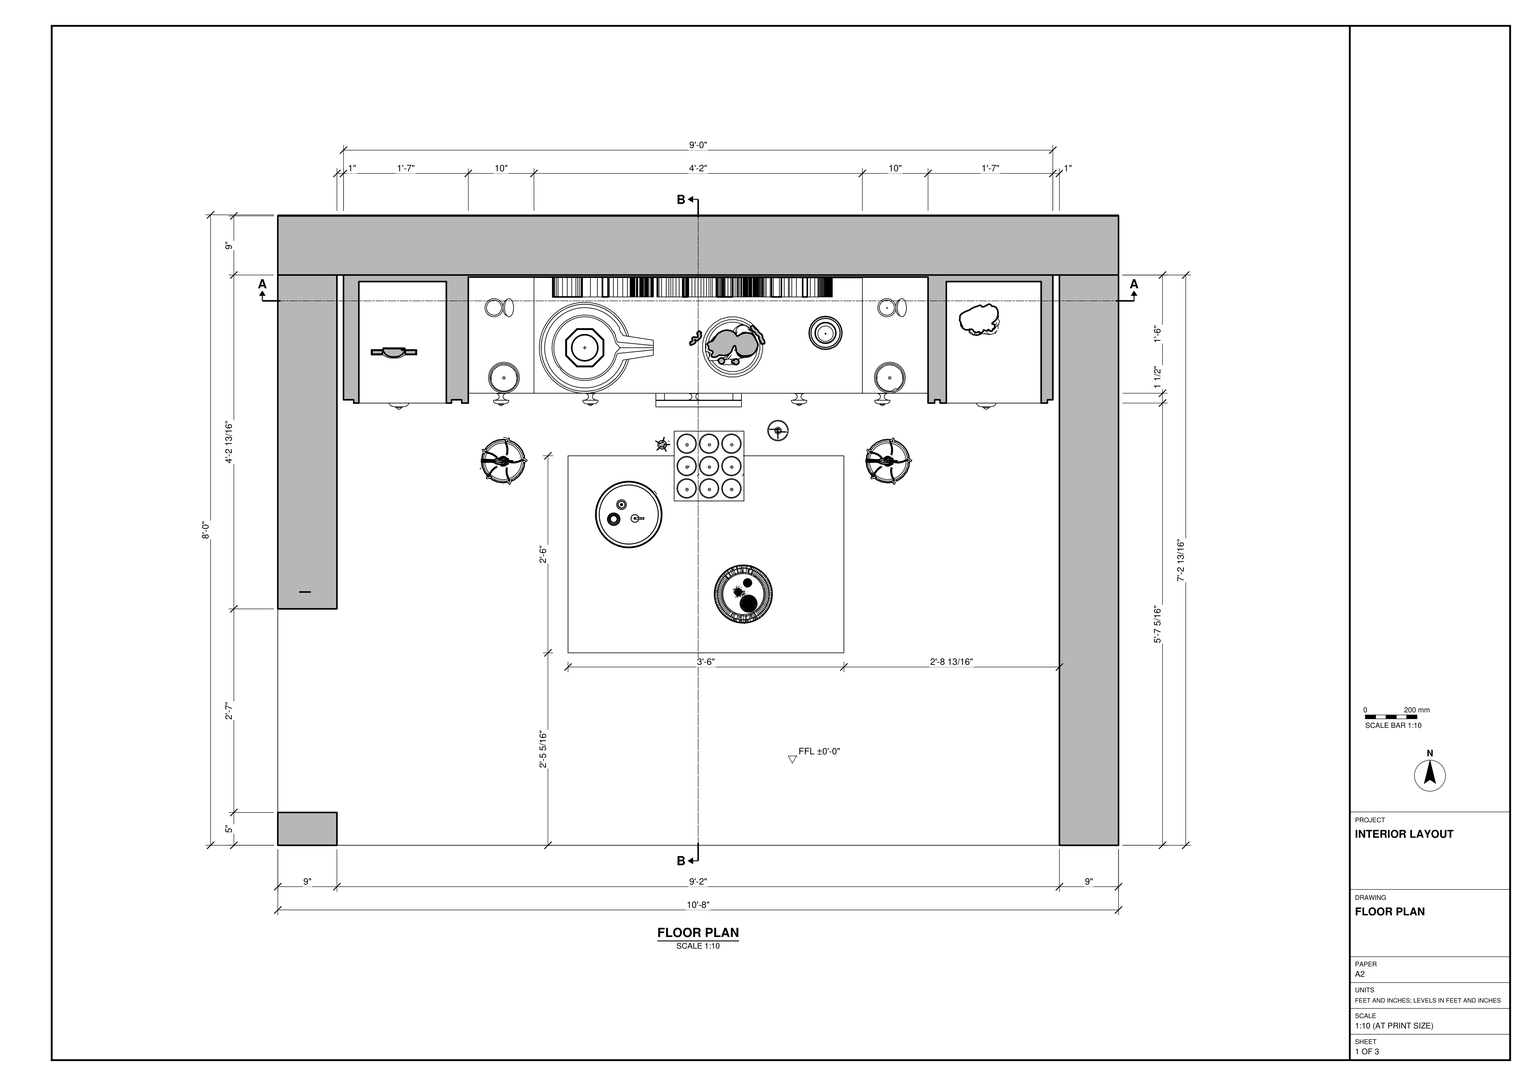
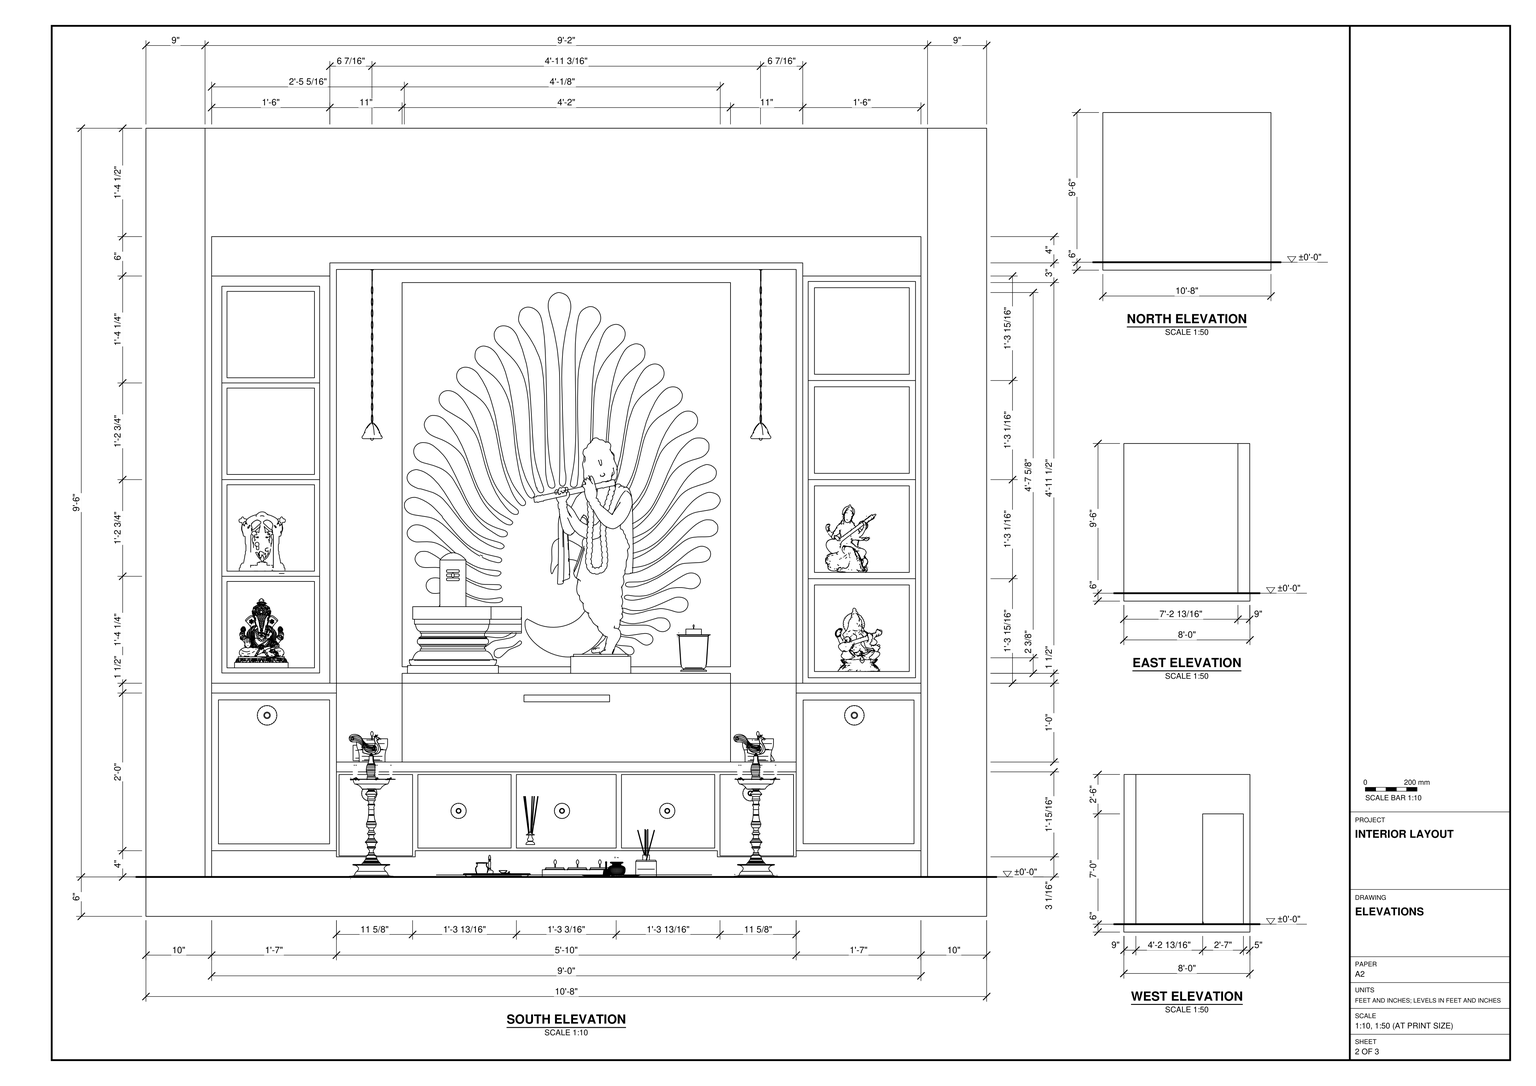
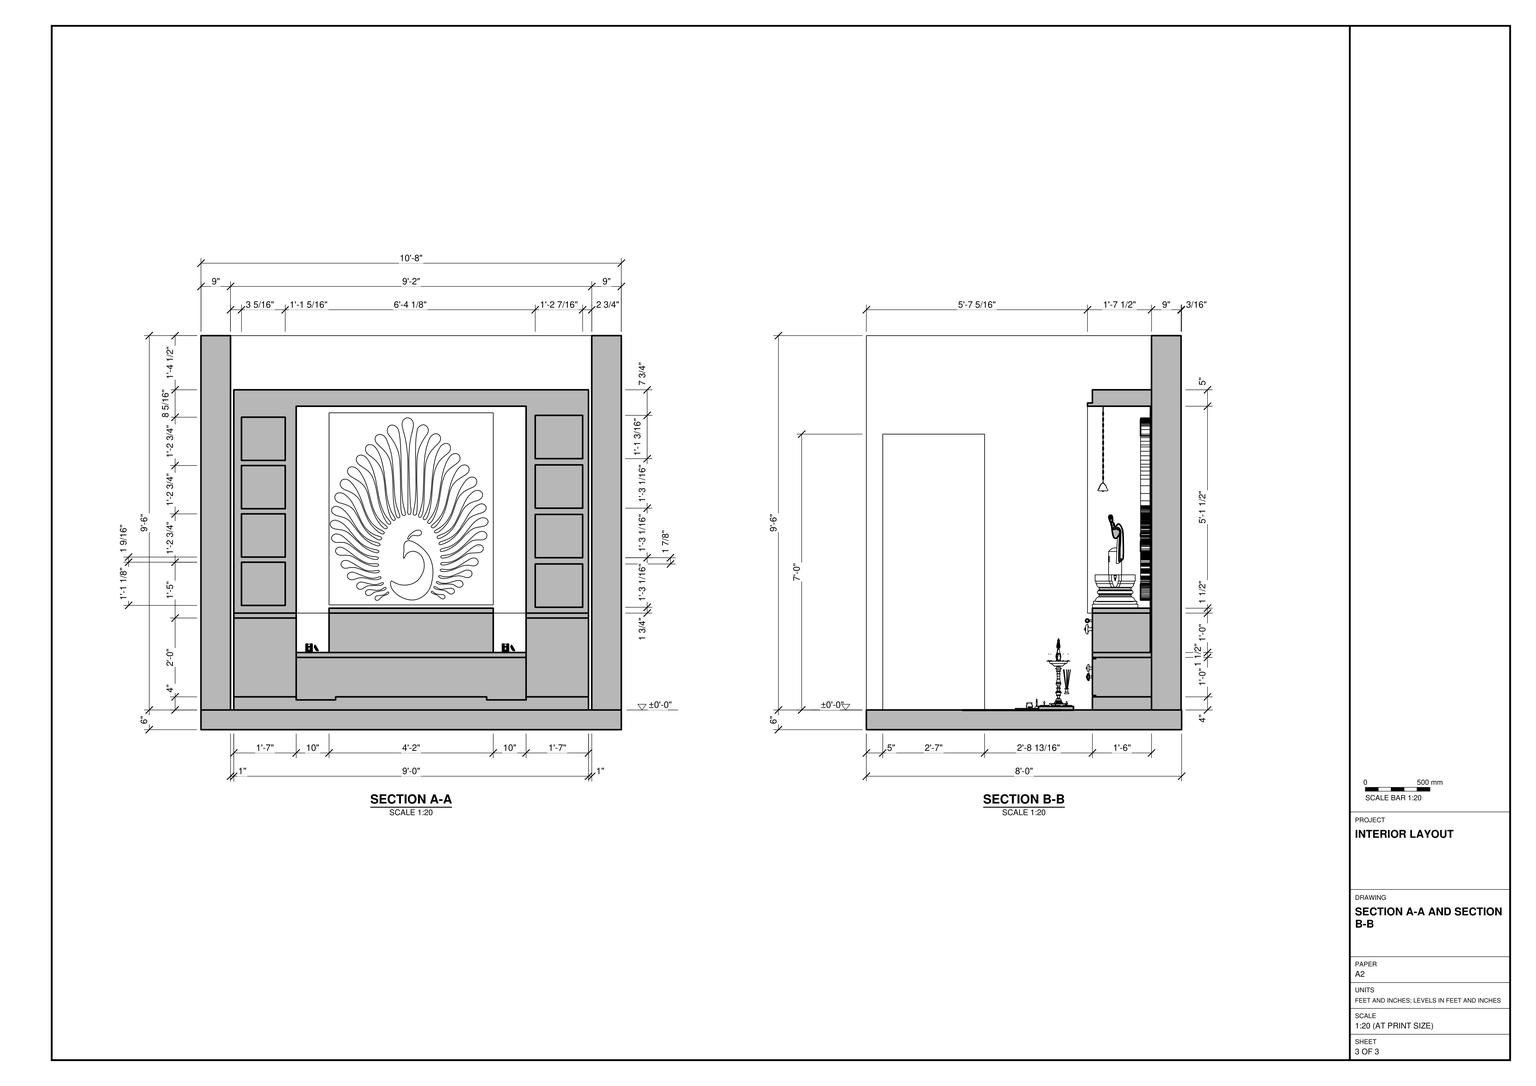
Build the prayer room in SketchUp from task_files/diagram_01.pdf. Work in feet and inches. Set the finished floor at ±0'-0". The room shell measures 10'-8" across the shrine wall and 8'-0" from front to back, with an overall height of 10'-0" from the underside of the slab. Model the 6" floor slab and the 9" walls. Leave the south side open as drawn and form the doorway near the south end of the west wall, retaining the short wall return beyond it.

Use the south elevation for the joinery fronts and the sections for their depths and changes in height. Build the 9'-0" shrine unit against the north wall. At each end, place a stack of display compartments above a lower cupboard. Between the cupboards, model the low storage run, the narrower raised display cabinet and the feature panel with its radiating motif. Include the headpiece that spans the display. Place figures on the raised surface and in the lower display compartments. Arrange the hanging ornaments, standing lamps and floor accessories using the plan and elevation together. Decor and loose items may be any suitable library components.

Keep the walls, floor slab and each furniture or joinery piece in separate groups or components, and use components for repeated parts. Save one SketchUp model as output_files/prayer_room_with_a_built_in_shrine.skp.

# SketchUp Ruby script. Lengths in inches.
U = 1.inch
M = Sketchup.active_model
def pt(a) = Geom::Point3d.new(a.map { |v| v * U })
def face(e, loops, mat)
  f = e.add_face(loops[0].map { |a| pt(a) })
  loops[1..].each { |l| e.add_face(l.map { |a| pt(a) }).erase! }
  f.material = f.back_material = mat if mat
  f
end
# faces: each face lists its corners as indices into pts; further lists are holes
def faces(e, pts, list, mat = nil) = list.each { |f| face(e, (f[0].is_a?(Array) ? f : [f]).map { |l| l.map { |i| pts[i] } }, mat) }
# xy, xz, yz: faces in a plane at the given z, y or x. An outline is a flat list of corners, or four numbers for a rectangle; further outlines are holes
def ring(l) = l.size == 4 ? [[l[0], l[1]], [l[2], l[1]], [l[2], l[3]], [l[0], l[3]]] : l.each_slice(2).to_a
def flat(e, list, mat, &to3) = list.each { |f| face(e, (f[0].is_a?(Array) ? f : [f]).map { |l| ring(l).map { |u, v| to3.(u, v) } }, mat) }
def xy(e, z, list, mat = nil) = flat(e, list, mat) { |x, y| [x, y, z] }
def xz(e, y, list, mat = nil) = flat(e, list, mat) { |x, z| [x, y, z] }
def yz(e, x, list, mat = nil) = flat(e, list, mat) { |y, z| [x, y, z] }
def lines(e, pts, list) = list.each { |a, b| e.add_line(pt(pts[a]), pt(pts[b])) }
# prism: a flat outline (further loops are holes) pulled along v
def prism(e, loops, v, mat = nil)
  f = face(e, loops, mat); d = Geom::Vector3d.new(v.map { |x| x * U })
  f.pushpull(f.normal.samedirection?(d) ? d.length : -d.length)
end
def box(e, o, s, mat = nil) = prism(e, [[o, [o[0] + s[0], o[1], o[2]], [o[0] + s[0], o[1] + s[1], o[2]], [o[0], o[1] + s[1], o[2]]]], [0, 0, s[2]], mat)
def at(x, y, z, deg = 0) = Geom::Transformation.translation(pt([x, y, z])) * Geom::Transformation.rotation(ORIGIN, Z_AXIS, deg.degrees)
def axes(o, x, y, z) = Geom::Transformation.new([*x, 0, *y, 0, *z, 0, *pt(o).to_a, 1])
def part(name) = M.definitions.add(name)
# library, detail: a bought-in or finely detailed component or shape, given as its bounding box
def library(name, o, s) = part(name).tap { |d| box(d.entities, o, s) }
def detail(e, o, s) = box(e.add_group.entities, o, s)
def put(e, d, t, mat = nil) = e.add_instance(d, t).tap { |i| i.material = mat if mat }
def group(e, t, mat = nil) = e.add_group.tap { |g| g.transformation = t; g.material = mat if mat }.entities
root = M.entities
M.materials.add("1795 AP 8578 CALAMINE").color = [220, 189, 165]
M.materials.add("1890 AP 0R08 ROSE PETAL").color = [217, 196, 185]
M.materials.add("2127 AP  X184 Madras Green-I").color = [32, 130, 100]
M.materials.add("Alphonsine+Classic+Style+Floral+Rug").color = [180, 185, 188]
M.materials.add("[0111_SlateGray]").color = [112, 128, 144]
M.materials.add("[Carrera Marble]").color = [206, 206, 206]
M.materials["[Carrera Marble]"].alpha = 0.93
M.materials.add("[Color B01]").color = [255, 216, 204]
M.materials.add("[Color C02]").color = [255, 204, 153]
M.materials.add("[Color C04]").color = [255, 153, 50]
M.materials.add("[Color E01]").color = [255, 255, 204]
M.materials.add("[Color M07]").color = [58, 58, 58]
M.materials.add("[Concrete Tile]").color = [201, 188, 162]
M.materials["[Concrete Tile]"].alpha = 0.93
M.materials.add("[Wood Cherry Original]2").color = [152, 86, 42]
M.materials.add("[Wood_Bamboo_Medium]1").color = [102, 17, 15]
c1 = library("Cabinet Knob",[0,0,0],[1.5,1.22,1.5])
c2 = library("d2b78a698ddc5cc256559ea918d5c8eb.dwg",[2.05,11.56,0],[44.08,53.19,3])
c3 = part("tubular wardrobe handle")
g1 = group(c3.entities,at(0,0,0),"[Color B01]")
xy(g1,0,[[0.197,0,0.591,0.984],[0.197,8.858,0.591,9.843]])
xy(g1,0.844,[[0.197,0.984,0.591,8.858]])
xz(g1,0,[[0.197,0,0.591,0,0.591,0.844,0.536,0.814,0.436,0.79,0.333,0.792,0.235,0.821,0.197,0.844],[0.436,0.79,0.536,0.814,0.591,0.844,0.626,0.863,0.7,0.934,0.754,1.022,0.783,1.121,0.784,1.181,0.785,1.223,0.761,1.323,0.712,1.413,0.641,1.488,0.553,1.541,0.454,1.57,0.351,1.573,0.252,1.548,0.161,1.499,0.087,1.428,0.034,1.34,0.005,1.242,0.003,1.181,0.002,1.139,0.027,1.039,0.076,0.949,0.147,0.874,0.197,0.844,0.235,0.821,0.333,0.792]])
xz(g1,0.984,[[0.197,0,0.591,0.844]])
xz(g1,8.858,[[0.197,0,0.591,0.844]])
xz(g1,9.843,[[0.197,0,0.197,0.844,0.235,0.821,0.333,0.792,0.436,0.79,0.536,0.814,0.591,0.844,0.591,0],[0.436,0.79,0.333,0.792,0.235,0.821,0.197,0.844,0.147,0.874,0.076,0.949,0.027,1.039,0.002,1.139,0.005,1.242,0.034,1.34,0.087,1.428,0.161,1.499,0.252,1.548,0.351,1.573,0.454,1.57,0.553,1.541,0.641,1.488,0.712,1.413,0.761,1.323,0.785,1.223,0.783,1.121,0.754,1.022,0.7,0.934,0.626,0.863,0.591,0.844,0.536,0.814]])
yz(g1,0.197,[[0,0,0.984,0.844],[8.858,0,9.843,0.844]])
yz(g1,0.591,[[0,0,0.984,0.844],[8.858,0,9.843,0.844]])
p = [[0.147,9.843,0.874],[0.197,9.843,0.844],[0.197,8.858,0.844],[0.197,0.984,0.844],[0.197,0,0.844],[0.147,0,0.874],
  [0.235,0,0.821],[0.235,9.843,0.821],[0.333,0,0.792],[0.333,9.843,0.792],[0.436,0,0.79],[0.436,9.843,0.79],
  [0.536,0,0.814],[0.536,9.843,0.814],[0.591,0,0.844],[0.591,9.843,0.844],[0.591,8.858,0.844],[0.591,0.984,0.844],
  [0.626,0,0.863],[0.626,9.843,0.863],[0.076,0,0.949],[0.027,0,1.039],[0.027,9.843,1.039],[0.076,9.843,0.949],
  [0.7,0,0.934],[0.7,9.843,0.934],[0.754,0,1.022],[0.754,9.843,1.022],[0.002,0,1.139],[0.002,9.843,1.139],
  [0.783,0,1.121],[0.783,9.843,1.121],[0.003,0,1.181],[0.005,0,1.242],[0.005,9.843,1.242],[0.785,0,1.223],
  [0.784,0,1.181],[0.785,9.843,1.223],[0.034,0,1.34],[0.034,9.843,1.34],[0.761,0,1.323],[0.761,9.843,1.323],
  [0.087,0,1.428],[0.087,9.843,1.428],[0.712,0,1.413],[0.712,9.843,1.413],[0.161,0,1.499],[0.161,9.843,1.499],
  [0.641,0,1.488],[0.641,9.843,1.488],[0.252,0,1.548],[0.252,9.843,1.548],[0.351,0,1.573],[0.351,9.843,1.573],
  [0.454,0,1.57],[0.553,0,1.541],[0.553,9.843,1.541],[0.454,9.843,1.57],[0.787,0,1.181],[0,0,1.181]]
faces(g1,p,[[0,1,2,3,4,5],[6,4,3,2,1,7],[8,6,7,9],[10,8,9,11],[12,10,11,13],[14,12,13,15,16,17],[18,14,17,16,15,19],[20,21,22,23],
  [5,20,23,0],[24,18,19,25],[26,24,25,27],[21,28,29,22],[30,26,27,31],[28,32,33,34,29],[35,36,30,31,37],[33,38,39,34],
  [40,35,37,41],[38,42,43,39],[44,40,41,45],[42,46,47,43],[48,44,45,49],[46,50,51,47],[50,52,53,51],[54,55,56,57],
  [55,48,49,56],[52,54,57,53]])
lines(g1,p,[[58,36],[59,32]])
c4 = part("Component\#32")
xy(c4.entities,0,[[0,-1.73,116.69,79.11]],"Alphonsine+Classic+Style+Floral+Rug")
xy(c4.entities,0.16,[[0.04,-1.6875,0.05,-1.68,0.05,79.06,0.04,79.07],[0.04,-1.6875,116.65,-1.6875,116.64,-1.68,0.05,-1.68],[116.65,-1.6875,116.65,79.07,116.64,79.06,116.64,-1.68],[0.05,79.06,116.64,79.06,116.65,79.07,0.04,79.07]],"Alphonsine+Classic+Style+Floral+Rug")
xy(c4.entities,0.17,[[0.07,-1.67,0.08,-1.65,0.08,79.03,0.07,79.04],[0.07,-1.67,116.625,-1.67,116.61,-1.65,0.08,-1.65],[116.625,-1.67,116.625,79.04,116.61,79.03,116.61,-1.65],[0.08,-1.65,116.61,79.03],[0.08,79.03,116.61,79.03,116.625,79.04,0.07,79.04]],"Alphonsine+Classic+Style+Floral+Rug")
xz(c4.entities,-1.73,[[0,0,116.69,0.09],[0,0.09,116.69,0.1],[0,0.1,116.69,0.1,116.6875,0.11,0,0.11]],"Alphonsine+Classic+Style+Floral+Rug")
xz(c4.entities,-1.72,[[0.01,0.125,116.68,0.125,116.68,0.13,0.02,0.13]],"Alphonsine+Classic+Style+Floral+Rug")
xz(c4.entities,79.1,[[0.01,0.125,0.02,0.13,116.68,0.13,116.68,0.125]],"Alphonsine+Classic+Style+Floral+Rug")
xz(c4.entities,79.11,[[0,0,116.69,0.09],[0,0.09,116.69,0.1],[0,0.1,0,0.11,116.6875,0.11,116.69,0.1]],"Alphonsine+Classic+Style+Floral+Rug")
yz(c4.entities,0,[[-1.73,0,79.11,0.09],[-1.73,0.09,79.11,0.1],[-1.73,0.1,79.11,0.11]],"Alphonsine+Classic+Style+Floral+Rug")
yz(c4.entities,0.02,[[-1.72,0.13,-1.71,0.14,79.09,0.14,79.1,0.13]],"Alphonsine+Classic+Style+Floral+Rug")
yz(c4.entities,116.68,[[-1.72,0.125,79.1,0.13]],"Alphonsine+Classic+Style+Floral+Rug")
yz(c4.entities,116.69,[[-1.73,0,79.11,0.09],[-1.73,0.09,79.11,0.1]],"Alphonsine+Classic+Style+Floral+Rug")
p = [[0.03,-1.7,0.15],[0.03,79.08,0.15],[0.02,79.09,0.14],[0.02,-1.71,0.14],[0.02,-1.72,0.13],[0.02,79.1,0.13],
  [0.01,79.1,0.125],[0.01,-1.72,0.125],[0,79.11,0.11],[0,-1.73,0.11],[116.66,-1.7,0.15],[116.67,-1.71,0.14],
  [116.68,-1.72,0.13],[116.68,-1.72,0.125],[116.6875,-1.73,0.11],[116.66,79.08,0.15],[116.67,79.09,0.14],[116.68,79.1,0.13],
  [116.68,79.1,0.125],[116.6875,79.11,0.11],[116.69,-1.73,0.1],[116.69,79.11,0.1],[0.04,-1.6875,0.16],[0.04,79.07,0.16],
  [116.65,-1.6875,0.16],[0.07,-1.67,0.17],[0.07,79.04,0.17],[0.05,79.06,0.16],[0.05,-1.68,0.16],[116.625,-1.67,0.17],
  [116.64,-1.68,0.16],[116.625,79.04,0.17],[116.64,79.06,0.16],[116.65,79.07,0.16]]
faces(c4.entities,p,[[0,1,2,3],[4,5,6,7],[7,6,8,9],[10,0,3,11],[11,3,4,12],[13,7,9,14],[15,10,11,16],[16,11,12,17],
  [18,13,14,19],[19,14,20,21],[1,15,16,2],[2,16,17,5],[6,18,19,8],[22,23,1,0],[24,22,0,10],[25,26,27,28],
  [29,25,28,30],[31,29,30,32],[33,24,10,15],[26,31,32,27],[23,33,15,1]],"Alphonsine+Classic+Style+Floral+Rug")
c5 = library("Votive candle",[0,0,0],[4.72,4.72,4.68])
c6 = library("Candle in holder",[0,0,0],[10.22,10.22,14.1875])
c7 = library("Saraswati idol",[-87.41,-75.68,0],[174.76,151.36,236.66])
c8 = library("Saraswati idol\#1",[0,0,0],[4.6,2.875,6.11])
c9 = library("venkateswara idol",[-15.36,-3.54,-19.6],[30.71,6.93,39.28])
c10 = library("Ganesha+-+An+Do+Giao",[8.43,-11.04,-0.14],[9.49,5.78,12.28])
c11 = part("d2")
xy(c11.entities,0,[[0,0,36,1.6]],"[Wood_Bamboo_Medium]1")
xy(c11.entities,72,[[0,0,36,1.6]],"[Wood_Bamboo_Medium]1")
yz(c11.entities,0,[[0,0,1.6,72]],"[Wood_Bamboo_Medium]1")
yz(c11.entities,36,[[0,0,1.6,72]],"[Wood_Bamboo_Medium]1")
c12 = library("pooja peacock diya",[491.62,2024.19,120],[8.72,8.65,21.71])
c13 = library("Group\#30",[-1.1875,-5.17,0],[15.05,16.41,31.1])
c14 = library("Group\#39",[0,0,0],[3.08,3.08,26.03])
c15 = library("Group\#41",[0,0,0],[8.88,8.88,3])
c16 = library("Group\#53",[0,0,0],[3.15,3.15,7.24])
c17 = library("Group\#55",[0,0,-0.2],[4.36,2.76,2.59])
c18 = library("Group\#57",[0,0,0],[10.63,10.63,2.71])
c19 = library("Group\#73",[14.35,14.41,-4],[60,59.88,92])
c20 = library("Group\#76",[-0.24,-0.75,0],[29.53,4.51,16.375])
c21 = library("Group\#75",[0,0,0],[262.22,209.17,100.13])
c22 = library("Group\#78",[-0.1,-0.1,0],[12.2,11.97,39.96])
c23 = library("Group\#86",[0,0,0],[134.16,133.89,43.06])
put(root,c1,axes([19.94,66.4,29.11],[-2,0,0],[0,2,0],[0,0,2]))
put(root,c1,axes([109.36,66.4,29.11],[-2,0,0],[0,2,0],[0,0,2]))
put(root,c1,axes([35.17,66.93,17.57],[-1.56,0,0],[0,1.56,0],[0,0,1.56]))
put(root,c1,axes([93.21,66.93,17.57],[-1.56,0,0],[0,1.56,0],[0,0,1.56]))
put(root,c1,axes([48.77,66.93,14.89],[-1.56,0,0],[0,1.56,0],[0,0,1.56]))
put(root,c1,axes([80.54,66.93,14.89],[-1.56,0,0],[0,1.56,0],[0,0,1.56]))
put(root,c2,axes([37.1,86.46,27.28],[1.09138,0,0],[0,0,1.04557],[0,-0.99,0]),"2127 AP  X184 Madras Green-I")
put(root,c1,axes([64.52,66.93,14.89],[-1.56,0,0],[0,1.56,0],[0,0,1.56]))
put(root,c3,axes([70.59,68.83,32.66],[0,0,1.32422],[-1.32422,0,0],[0,-1.32422,0]))
put(root,c4,axes([44.1875,29.95,5.875],[0.35992,0,0],[0,0.37109,0],[0,0,1]))
put(root,c5,at(90.82,68.83,23.5))
put(root,c6,axes([80.83,75.47,37.3125],[0.5,0,0],[0,0.5,0],[0,0,0.5]))
put(root,c5,at(32.07,68.83,23.5))
put(root,c7,axes([108.5,74.73,37.28],[0.04079,0,0],[0,0.04079,0],[0,0,0.04079]))
put(root,c8,axes([103.75,76.94,52.37],[1.67304,0.23513,0],[-0.23513,1.67304,0],[0,0,1.68948]))
put(root,c9,axes([17.6875,74.99,57.07],[0.23,0,0],[0,0.23,0],[0,0,0.23]))
put(root,c10,axes([6.24,80.36,37.96],[0.86,0,0],[0,0.86,0],[0,0,0.86]))
put(root,c11,axes([4.9375,5,0],[0,0.93245,0],[-1,0,0],[0,0,1.25]))
put(root,c12,at(-461.625,-1969.84,-114))
put(root,c12,at(-403.0625,-1969.84,-114))
g2 = group(root,at(10,24,0),"[Concrete Tile]")
box(g2,[-10,-24,0],[128,96,6])
g3 = group(root,at(10,86.83,6),"1795 AP 8578 CALAMINE")
box(g3,[-10,0,0],[128,9,114])
g4 = group(root,at(10,70.83,6),"[Carrera Marble]")
prism(g4,[[[108,16,0],[0,16,0],[0,16,4],[19,16,4],[19,16,3.0625],[31,16,3.0625],[31,16,4],[77,16,4],[77,16,3.0625],[89,16,3.0625],[89,16,4],[108,16,4]]],[0,-18,0])
g5 = group(root,at(10,84.83,35.5),"[Wood Cherry Original]2")
xy(g5,0,[[18,-17.5,18,-17,0,-17,0,2,108,2,108,-17,90,-17,90,-17.5,89,-17.5,89,1.6875,19,1.6875,19,-17.5]])
xy(g5,0.83,[[90.83,-17.5,107.17,-17]])
xy(g5,1.56,[[1.56,-17.5,16.44,-17]])
xy(g5,1.78,[[91.78,-17.5,106.22,1]])
xy(g5,2.34,[[2.34,-17.5,15.66,1]])
xy(g5,14.96,[[91.78,-17.5,106.22,1]])
xy(g5,15.49,[[2.34,-17.5,15.66,1]])
xy(g5,16.87,[[91.78,-17.5,106.22,1]])
xy(g5,17.0625,[[2.34,-17.5,15.66,1]])
xy(g5,30.05,[[91.78,-17.5,106.22,1]])
xy(g5,30.22,[[2.34,-17.5,15.66,1]])
xy(g5,31.78,[[2.34,-17.5,15.66,1]])
xy(g5,31.95,[[91.78,-17.5,106.22,1]])
xy(g5,44.9375,[[2.34,-17.5,15.66,1]])
xy(g5,45.13,[[91.78,-17.5,106.22,1]])
xy(g5,46.51,[[2.34,-17.5,15.66,1]])
xy(g5,47.04,[[91.78,-17.5,106.22,1]])
xy(g5,59.66,[[2.34,-17.5,15.66,1]])
xy(g5,60.22,[[91.78,-17.5,106.22,1]])
xy(g5,60.44,[[1.56,-17.5,16.44,-17]])
xy(g5,61.17,[[90.83,-17.5,107.17,-17]])
xy(g5,62,[[0,-17,18,-16],[90,-17,108,-16]])
xy(g5,63,[[19,-17.5,89,1.6875]])
xy(g5,64,[[18,-17.5,90,-16]])
xy(g5,68,[[0,-16,108,2]])
xz(g5,-17.5,[[18,0,19,0,19,63,89,63,89,0,90,0,90,64,18,64],[[90.83,0.83,107.17,15.91],[91.78,1.78,106.22,14.96]],[[1.56,1.56,16.44,16.28],[2.34,2.34,15.66,15.49]],[[90.83,15.91,107.17,31],[91.78,16.87,106.22,30.05]],[[1.56,16.28,16.44,31],[2.34,17.0625,15.66,30.22]],
  [[1.56,31,16.44,45.72],[2.34,31.78,15.66,44.9375]],[[90.83,31,107.17,46.09],[91.78,31.95,106.22,45.13]],[[1.56,45.72,16.44,60.44],[2.34,46.51,15.66,59.66]],[[90.83,46.09,107.17,61.17],[91.78,47.04,106.22,60.22]]])
xz(g5,-17,[[[0,0,18,62],[1.56,1.56,16.44,60.44]],[[90,0,108,62],[90.83,0.83,107.17,61.17]]])
xz(g5,-16,[[0,62,18,62,18,64,90,64,90,62,108,62,108,68,0,68]])
xz(g5,1,[[91.78,1.78,106.22,14.96],[2.34,2.34,15.66,15.49],[91.78,16.87,106.22,30.05],[2.34,17.0625,15.66,30.22],[2.34,31.78,15.66,44.9375],
  [91.78,31.95,106.22,45.13],[2.34,46.51,15.66,59.66],[91.78,47.04,106.22,60.22]])
xz(g5,1.6875,[[19,0,89,63]])
xz(g5,2,[[0,0,108,68]])
yz(g5,0,[[-17,0,-17,62,-16,62,-16,68,2,68,2,0]])
yz(g5,1.56,[[-17.5,1.56,-17,16.28],[-17.5,16.28,-17,31],[-17.5,31,-17,45.72],[-17.5,45.72,-17,60.44]])
yz(g5,2.34,[[-17.5,2.34,1,15.49],[-17.5,17.0625,1,30.22],[-17.5,31.78,1,44.9375],[-17.5,46.51,1,59.66]])
yz(g5,15.66,[[-17.5,2.34,1,15.49],[-17.5,17.0625,1,30.22],[-17.5,31.78,1,44.9375],[-17.5,46.51,1,59.66]])
yz(g5,16.44,[[-17.5,1.56,-17,16.28],[-17.5,16.28,-17,31],[-17.5,31,-17,45.72],[-17.5,45.72,-17,60.44]])
yz(g5,18,[[-17.5,0,-17,62],[-17.5,62,-16,64]])
yz(g5,19,[[-17.5,0,1.6875,63]])
yz(g5,89,[[-17.5,0,1.6875,63]])
yz(g5,90,[[-17.5,0,-17,62],[-17.5,62,-16,64]])
yz(g5,90.83,[[-17.5,0.83,-17,15.91],[-17.5,15.91,-17,31],[-17.5,31,-17,46.09],[-17.5,46.09,-17,61.17]])
yz(g5,91.78,[[-17.5,1.78,1,14.96],[-17.5,16.87,1,30.05],[-17.5,31.95,1,45.13],[-17.5,47.04,1,60.22]])
yz(g5,106.22,[[-17.5,1.78,1,14.96],[-17.5,16.87,1,30.05],[-17.5,31.95,1,45.13],[-17.5,47.04,1,60.22]])
yz(g5,107.17,[[-17.5,0.83,-17,15.91],[-17.5,15.91,-17,31],[-17.5,31,-17,46.09],[-17.5,46.09,-17,61.17]])
yz(g5,108,[[-17,0,2,0,2,68,-16,68,-16,62,-17,62]])
p = [[79,1.625,61],[29,1.6875,61],[29,1.6875,2.5],[79,1.625,2.5]]
faces(g5,p,[[0,1,2,3]],"[Wood Cherry Original]2")
g6 = group(root,at(10,68.83,10),"1890 AP 0R08 ROSE PETAL")
xy(g6,0,[[0,1,19,18]])
xy(g6,1.04,[[1.04,0,17.96,1]])
xy(g6,22.96,[[1.04,0,17.96,1]])
xy(g6,24,[[0,1,19,18]])
xz(g6,0,[[1.04,1.04,17.96,22.96]])
xz(g6,1,[[[0,0,19,24],[1.04,1.04,17.96,22.96]]])
xz(g6,18,[[0,0,19,24]])
yz(g6,0,[[1,0,18,24]])
yz(g6,1.04,[[0,1.04,1,22.96]])
yz(g6,17.96,[[0,1.04,1,22.96]])
yz(g6,19,[[1,0,18,24]])
g7 = group(root,at(99,68.83,10),"1890 AP 0R08 ROSE PETAL")
xy(g7,0,[[0,1,19,18]])
xy(g7,1.0625,[[1.0625,0,17.9375,1]])
xy(g7,22.9375,[[1.0625,0,17.9375,1]])
xy(g7,24,[[0,1,19,18]])
xz(g7,0,[[1.0625,1.0625,17.9375,22.9375]])
xz(g7,1,[[[0,0,19,24],[1.0625,1.0625,17.9375,22.9375]]])
xz(g7,18,[[0,0,19,24]])
yz(g7,0,[[1,0,18,24]])
yz(g7,1.0625,[[0,1.0625,1,22.9375]])
yz(g7,17.9375,[[0,1.0625,1,22.9375]])
yz(g7,19,[[1,0,18,24]])
g8 = group(root,at(29,68.83,10),"1890 AP 0R08 ROSE PETAL")
xy(g8,-0.9375,[[0,1,12,18],[58,1,70,18]])
xy(g8,-0.79,[[0.4,0,11.6,1],[58.4,0,69.6,1]])
xy(g8,0,[[12,1,58,18]])
xy(g8,0.4,[[12.4,0,26.6,1],[27.4,0,42.6,1],[43.4,0,57.6,1]])
xy(g8,11.6,[[0.4,0,11.6,1],[12.4,0,26.6,1],[27.4,0,42.6,1],[43.4,0,57.6,1],[58.4,0,69.6,1]])
xy(g8,12,[[0,1,70,18]])
xz(g8,0,[[0.4,-0.79,11.6,11.6],[58.4,-0.79,69.6,11.6],[12.4,0.4,26.6,11.6],[27.4,0.4,42.6,11.6],[43.4,0.4,57.6,11.6]])
xz(g8,1,[[[0,-0.9375,12,-0.9375,12,0,58,0,58,-0.9375,70,-0.9375,70,12,0,12],[27.4,0.4,42.6,11.6],[43.4,0.4,57.6,11.6],[12.4,0.4,26.6,11.6],[0.4,-0.79,11.6,11.6],[58.4,-0.79,69.6,11.6]]])
xz(g8,18,[[0,-0.9375,0,12,70,12,70,-0.9375,58,-0.9375,58,0,12,0,12,-0.9375]])
yz(g8,0,[[1,-0.9375,18,12]])
yz(g8,0.4,[[0,-0.79,1,11.6]])
yz(g8,11.6,[[0,-0.79,1,11.6]])
yz(g8,12,[[1,-0.9375,18,0]])
yz(g8,12.4,[[0,0.4,1,11.6]])
yz(g8,26.6,[[0,0.4,1,11.6]])
yz(g8,27.4,[[0,0.4,1,11.6]])
yz(g8,42.6,[[0,0.4,1,11.6]])
yz(g8,43.4,[[0,0.4,1,11.6]])
yz(g8,57.6,[[0,0.4,1,11.6]])
yz(g8,58,[[1,-0.9375,18,0]])
yz(g8,58.4,[[0,-0.79,1,11.6]])
yz(g8,69.6,[[0,-0.79,1,11.6]])
yz(g8,70,[[1,-0.9375,18,12]])
g9 = group(root,at(41,68.46,23.5),"1890 AP 0R08 ROSE PETAL")
box(g9,[-2,0.375,0],[50,17.625,12])
g10 = group(root,at(29,68.83,22),"1890 AP 0R08 ROSE PETAL")
box(g10,[0,0,0],[70,18,1.5])
g11 = group(root,at(41,68.46,35.5),"1890 AP 0R08 ROSE PETAL")
box(g11,[-2,0.375,0],[50,17.625,1.5])
g12 = group(root,at(10,68.83,34),"1890 AP 0R08 ROSE PETAL")
box(g12,[0,0,0],[19,18,1.5])
g13 = group(root,at(99,68.83,34),"1890 AP 0R08 ROSE PETAL")
box(g13,[0,0,0],[19,18,1.5])
put(root,c13,axes([74.34,80.47,37],[-1.16,0,0],[0,-1.16,0],[0,0,1.16]))
put(root,c14,at(32.89,70.48,72.47))
put(root,c14,at(92.07,70.48,72.47))
put(root,c15,at(66.43,33.82,6.04))
put(root,c16,at(74.57,61.57,6))
g14 = group(root,at(92.68,81.77,25.27))
xy(g14,0,[[0.116,0,0.168,0,0.168,0.067,0.132,0.067]],"[Color E01]")
xz(g14,0,[[0.116,0,0.168,0,0.116,0.128]],"[0111_SlateGray]")
xz(g14,0.067,[[0.132,0,0.132,0.128,0.168,0]],"[0111_SlateGray]")
p = [[0.116,0,0],[0.116,0,0.128],[0.112,0.001,0.134],[0.093,0.006,0.184],[0.078,0.009,0.236],[0.069,0.011,0.289],
  [0.067,0.012,0.343],[0.069,0.011,0.396],[0.078,0.009,0.45],[0.093,0.006,0.501],[0.112,0.001,0.551],[0.116,0,0.557],
  [0.116,0,0.685],[0.081,0.008,0.635],[0.052,0.015,0.581],[0.03,0.021,0.524],[0.013,0.025,0.465],[0.003,0.027,0.404],
  [0,0.028,0.343],[0.003,0.027,0.281],[0.013,0.025,0.22],[0.03,0.021,0.161],[0.052,0.015,0.104],[0.081,0.008,0.05],
  [0.168,0,0],[0.132,0.067,0.128],[0.168,0.067,0],[0.097,0.075,0.05],[0.132,0.067,0],[0.069,0.082,0.104],
  [0.046,0.088,0.161],[0.03,0.092,0.22],[0.02,0.094,0.281],[0.016,0.095,0.343],[0.02,0.094,0.404],[0.03,0.092,0.465],
  [0.046,0.088,0.524],[0.069,0.082,0.581],[0.097,0.075,0.635],[0.132,0.067,0.685],[0.132,0.067,0.557],[0.129,0.067,0.551],
  [0.109,0.072,0.501],[0.094,0.076,0.45],[0.086,0.078,0.396],[0.083,0.079,0.343],[0.086,0.078,0.289],[0.094,0.076,0.236],
  [0.109,0.072,0.184],[0.129,0.067,0.134]]
faces(g14,p,[[0,1,2,3,4,5,6,7,8,9,10,11,12,13,14,15,16,17,18,19,20,21,22,23],[24,25,1],[25,24,26],[0,23,27,28],[25,28,27,29,30,31,32,33,34,35,36,37,38,39,40,41,42,43,44,45,46,47,48,49],[22,21,30,29],[3,2,49,48],[23,22,29,27],
  [2,1,25,49],[21,20,31,30],[20,19,32,31],[5,4,47,46],[4,3,48,47],[19,18,33,32],[18,17,34,33],[6,5,46,45],
  [7,6,45,44],[17,16,35,34],[9,8,43,42],[8,7,44,43],[15,14,37,36],[16,15,36,35],[10,9,42,41],[14,13,38,37],
  [12,11,40,39],[13,12,39,38],[11,10,41,40]],"[0111_SlateGray]")
faces(g14,p,[[1,0,28,25]])
put(root,c17,at(91.35,80.48,23.7))
put(root,c18,at(60.34,52.43,5.92))
put(root,c17,at(31.54,80.48,23.7))
g15 = group(root,at(39.8125,68.83,37),"[Color M07]")
g16 = group(g15,at(3.98,3.99,9.04))
xy(g16,0,[[[1.76,0.09,0.09,1.76,0.09,4.11,1.76,5.78,4.11,5.78,5.78,4.11,5.78,1.76,4.11,0.09],[2.8125,0.95,3.0625,0.95,3.31,0.99,3.55,1.05,3.7,1.1,3.78,1.14,4,1.26,4.2,1.41,4.38,1.58,4.54,1.77,4.68,1.98,4.78,2.21,4.86,2.44,4.91,2.6875,4.92,2.9375,4.91,3.1875,4.86,3.43,4.78,3.67,4.68,3.89,4.54,4.1,4.38,4.3,4.2,4.47,4,4.61,3.78,4.73,3.55,4.83,3.31,4.89,3.0625,4.92,2.8125,4.92,2.5625,4.89,2.32,4.83,2.18,4.77,2.09,4.73,1.87,4.61,1.67,4.47,1.49,4.3,1.33,4.1,1.2,3.89,1.09,3.67,1.01,3.43,0.97,3.1875,0.95,2.9375,0.97,2.6875,1.01,2.44,1.09,2.21,1.2,1.98,1.33,1.77,1.49,1.58,1.67,1.41,1.87,1.26,2.09,1.14,2.32,1.05,2.5625,0.99]]])
xy(g16,0.13,[[[1.76,0.09,4.11,0.09,5.78,1.76,5.78,4.11,4.11,5.78,1.76,5.78,0.09,4.11,0.09,1.76],[1.8,0.1875,0.1875,1.8,0.1875,4.07,1.8,5.68,4.07,5.68,5.68,4.07,5.68,1.8,4.07,0.1875]]])
xy(g16,0.83,[[[1.76,0.09,0.09,1.76,0.09,4.11,1.76,5.78,4.11,5.78,5.78,4.11,5.78,1.76,4.11,0.09],[1.8,0.1875,4.07,0.1875,5.68,1.8,5.68,4.07,4.07,5.68,1.8,5.68,0.1875,4.07,0.1875,1.8]]])
xy(g16,0.98,[[[1.72,0,0,1.72,0,4.15,1.72,5.875,4.15,5.875,5.875,4.15,5.875,1.72,4.15,0],[1.76,0.09,4.11,0.09,5.78,1.76,5.78,4.11,4.11,5.78,1.76,5.78,0.09,4.11,0.09,1.76]]])
xy(g16,1.12,[[[1.72,0,4.15,0,5.875,1.72,5.875,4.15,4.15,5.875,1.72,5.875,0,4.15,0,1.72],[2.8125,0.95,2.5625,0.99,2.32,1.05,2.09,1.14,1.87,1.26,1.67,1.41,1.49,1.58,1.33,1.77,1.2,1.98,1.09,2.21,1.01,2.44,0.97,2.6875,0.95,2.9375,0.97,3.1875,1.01,3.43,1.09,3.67,1.2,3.89,1.33,4.1,1.49,4.3,1.67,4.47,1.87,4.61,2.09,4.73,2.32,4.83,2.5625,4.89,2.8125,4.92,3.0625,4.92,3.31,4.89,3.55,4.83,3.78,4.73,4,4.61,4.2,4.47,4.38,4.3,4.54,4.1,4.68,3.89,4.78,3.67,4.86,3.43,4.91,3.1875,4.92,2.9375,4.91,2.6875,4.86,2.44,4.78,2.21,4.68,1.98,4.54,1.77,4.38,1.58,4.2,1.41,4,1.26,3.78,1.14,3.55,1.05,3.31,0.99,3.0625,0.95]]])
xz(g16,0,[[1.72,0.98,4.15,1.12]])
xz(g16,0.09,[[1.76,0,4.11,0.13],[1.76,0.83,4.11,0.98]])
xz(g16,0.1875,[[1.8,0.13,4.07,0.83]])
xz(g16,0.95,[[2.8125,0,3.0625,1.12]])
xz(g16,4.92,[[2.8125,0,3.0625,1.12]])
xz(g16,5.68,[[1.8,0.13,4.07,0.83]])
xz(g16,5.78,[[1.76,0,4.11,0.13],[1.76,0.83,4.11,0.98]])
xz(g16,5.875,[[1.72,0.98,4.15,1.12]])
yz(g16,0,[[1.72,0.98,4.15,1.12]])
yz(g16,0.09,[[1.76,0,4.11,0.13],[1.76,0.83,4.11,0.98]])
yz(g16,0.1875,[[1.8,0.13,4.07,0.83]])
yz(g16,5.68,[[1.8,0.13,4.07,0.83]])
yz(g16,5.78,[[1.76,0,4.11,0.13],[1.76,0.83,4.11,0.98]])
yz(g16,5.875,[[1.72,0.98,4.15,1.12]])
p = [[1.76,0.09,0.13],[0.09,1.76,0.13],[0.09,1.76,0],[1.76,0.09,0],[5.78,1.76,0.13],[4.11,0.09,0.13],
  [4.11,0.09,0],[5.78,1.76,0],[2.09,1.14,1.12],[2.32,1.05,1.12],[2.32,1.05,0],[2.09,1.14,0],
  [2.5625,0.99,1.12],[2.5625,0.99,0],[2.8125,0.95,1.12],[2.8125,0.95,0],[3.0625,0.95,1.12],[3.31,0.99,1.12],
  [3.31,0.99,0],[3.0625,0.95,0],[3.55,1.05,1.12],[3.55,1.05,0],[3.78,1.14,1.12],[3.78,1.14,0],
  [3.7,1.1,0],[1.87,1.26,1.12],[1.87,1.26,0],[4,1.26,1.12],[4,1.26,0],[1.67,1.41,1.12],
  [1.67,1.41,0],[4.2,1.41,1.12],[4.2,1.41,0],[1.49,1.58,1.12],[1.49,1.58,0],[4.38,1.58,1.12],
  [4.38,1.58,0],[1.33,1.77,1.12],[1.33,1.77,0],[4.54,1.77,1.12],[4.54,1.77,0],[1.2,1.98,1.12],
  [1.2,1.98,0],[4.68,1.98,1.12],[4.68,1.98,0],[1.09,2.21,1.12],[1.09,2.21,0],[4.78,2.21,1.12],
  [4.78,2.21,0],[1.01,2.44,1.12],[1.01,2.44,0],[4.86,2.44,1.12],[4.86,2.44,0],[0.97,2.6875,1.12],
  [0.97,2.6875,0],[4.91,2.6875,1.12],[4.91,2.6875,0],[0.95,2.9375,1.12],[0.95,2.9375,0],[4.92,2.9375,1.12],
  [4.92,2.9375,0],[0.97,3.1875,1.12],[0.97,3.1875,0],[4.91,3.1875,1.12],[4.91,3.1875,0],[1.01,3.43,1.12],
  [1.01,3.43,0],[4.86,3.43,1.12],[4.86,3.43,0],[1.09,3.67,1.12],[1.09,3.67,0],[4.78,3.67,1.12],
  [4.78,3.67,0],[1.2,3.89,1.12],[1.2,3.89,0],[4.68,3.89,1.12],[4.68,3.89,0],[1.33,4.1,1.12],
  [1.33,4.1,0],[4.54,4.1,1.12],[4.54,4.1,0],[0.09,4.11,0.13],[1.76,5.78,0.13],[1.76,5.78,0],
  [0.09,4.11,0],[1.49,4.3,1.12],[1.49,4.3,0],[4.11,5.78,0.13],[5.78,4.11,0.13],[5.78,4.11,0],
  [4.11,5.78,0],[4.38,4.3,1.12],[4.38,4.3,0],[1.67,4.47,1.12],[1.67,4.47,0],[4.2,4.47,1.12],
  [4.2,4.47,0],[1.87,4.61,1.12],[1.87,4.61,0],[4,4.61,1.12],[4,4.61,0],[2.09,4.73,1.12],
  [2.09,4.73,0],[3.78,4.73,1.12],[3.78,4.73,0],[2.32,4.83,1.12],[2.18,4.77,0],[2.32,4.83,0],
  [3.55,4.83,1.12],[3.55,4.83,0],[2.5625,4.89,1.12],[2.5625,4.89,0],[3.31,4.89,1.12],[3.31,4.89,0],
  [2.8125,4.92,1.12],[2.8125,4.92,0],[3.0625,4.92,1.12],[3.0625,4.92,0],[1.8,0.1875,0.83],[0.1875,1.8,0.83],
  [0.1875,1.8,0.13],[1.8,0.1875,0.13],[5.68,1.8,0.83],[4.07,0.1875,0.83],[4.07,0.1875,0.13],[5.68,1.8,0.13],
  [0.1875,4.07,0.83],[1.8,5.68,0.83],[1.8,5.68,0.13],[0.1875,4.07,0.13],[4.07,5.68,0.83],[5.68,4.07,0.83],
  [5.68,4.07,0.13],[4.07,5.68,0.13],[1.76,0.09,0.98],[0.09,1.76,0.98],[0.09,1.76,0.83],[1.76,0.09,0.83],
  [5.78,1.76,0.98],[4.11,0.09,0.98],[4.11,0.09,0.83],[5.78,1.76,0.83],[0.09,4.11,0.98],[1.76,5.78,0.98],
  [1.76,5.78,0.83],[0.09,4.11,0.83],[4.11,5.78,0.98],[5.78,4.11,0.98],[5.78,4.11,0.83],[4.11,5.78,0.83],
  [1.72,0,1.12],[0,1.72,1.12],[0,1.72,0.98],[1.72,0,0.98],[5.875,1.72,1.12],[4.15,0,1.12],
  [4.15,0,0.98],[5.875,1.72,0.98],[0,4.15,1.12],[1.72,5.875,1.12],[1.72,5.875,0.98],[0,4.15,0.98],
  [4.15,5.875,1.12],[5.875,4.15,1.12],[5.875,4.15,0.98],[4.15,5.875,0.98],[0.1875,4.07,0]]
faces(g16,p,[[0,1,2,3],[4,5,6,7],[8,9,10,11],[9,12,13,10],[12,14,15,13],[16,17,18,19],[17,20,21,18],[20,22,23,24,21],
  [25,8,11,26],[22,27,28,23],[29,25,26,30],[27,31,32,28],[33,29,30,34],[31,35,36,32],[37,33,34,38],[35,39,40,36],
  [41,37,38,42],[39,43,44,40],[45,41,42,46],[43,47,48,44],[49,45,46,50],[47,51,52,48],[53,49,50,54],[51,55,56,52],
  [57,53,54,58],[55,59,60,56],[61,57,58,62],[59,63,64,60],[65,61,62,66],[63,67,68,64],[69,65,66,70],[67,71,72,68],
  [73,69,70,74],[71,75,76,72],[77,73,74,78],[75,79,80,76],[81,82,83,84],[85,77,78,86],[87,88,89,90],[79,91,92,80],
  [93,85,86,94],[91,95,96,92],[97,93,94,98],[95,99,100,96],[101,97,98,102],[99,103,104,100],[105,101,102,106,107],[103,108,109,104],
  [110,105,107,111],[108,112,113,109],[114,110,111,115],[112,116,117,113],[118,119,120,121],[122,123,124,125],[126,127,128,129],[130,131,132,133],
  [134,135,136,137],[138,139,140,141],[142,143,144,145],[146,147,148,149],[150,151,152,153],[154,155,156,157],[158,159,160,161],[162,163,164,165]])
lines(g16,p,[[129,166]])
put(g15,c19,axes([3.98,3.99,9.45],[0.06622,0,0],[0,0.06622,0],[0,0,0.10144]))
put(g15,c20,axes([5.96,4.94,14.11],[0.06622,0,0],[0,0.06622,0],[0,0,0.10144]),"[Color C04]")
put(g15,c21,axes([0,0,0],[0.06622,0,0],[0,0.06622,0],[0,0,0.10144]))
put(root,c22,axes([57.5,59.98,10.93],[0.1837,0,0],[0,0.1837,0],[0,0,0.1837]))
put(root,c23,axes([48.34,45.28,6.04],[0.0759,0,0],[0,0.0759,0],[0,0,0.0759]),"[Color C02]")
g17 = group(root,at(0,0,6),"1795 AP 8578 CALAMINE")
prism(g17,[[[0,86.83,114],[0,86.83,0],[0,36,0],[0,36,84],[0,5,84],[0,5,0],[0,0,0],[0,0,114]]],[9,0,0])
g18 = group(root,at(119,0,6),"1795 AP 8578 CALAMINE")
box(g18,[0,0,0],[9,86.83,114])
